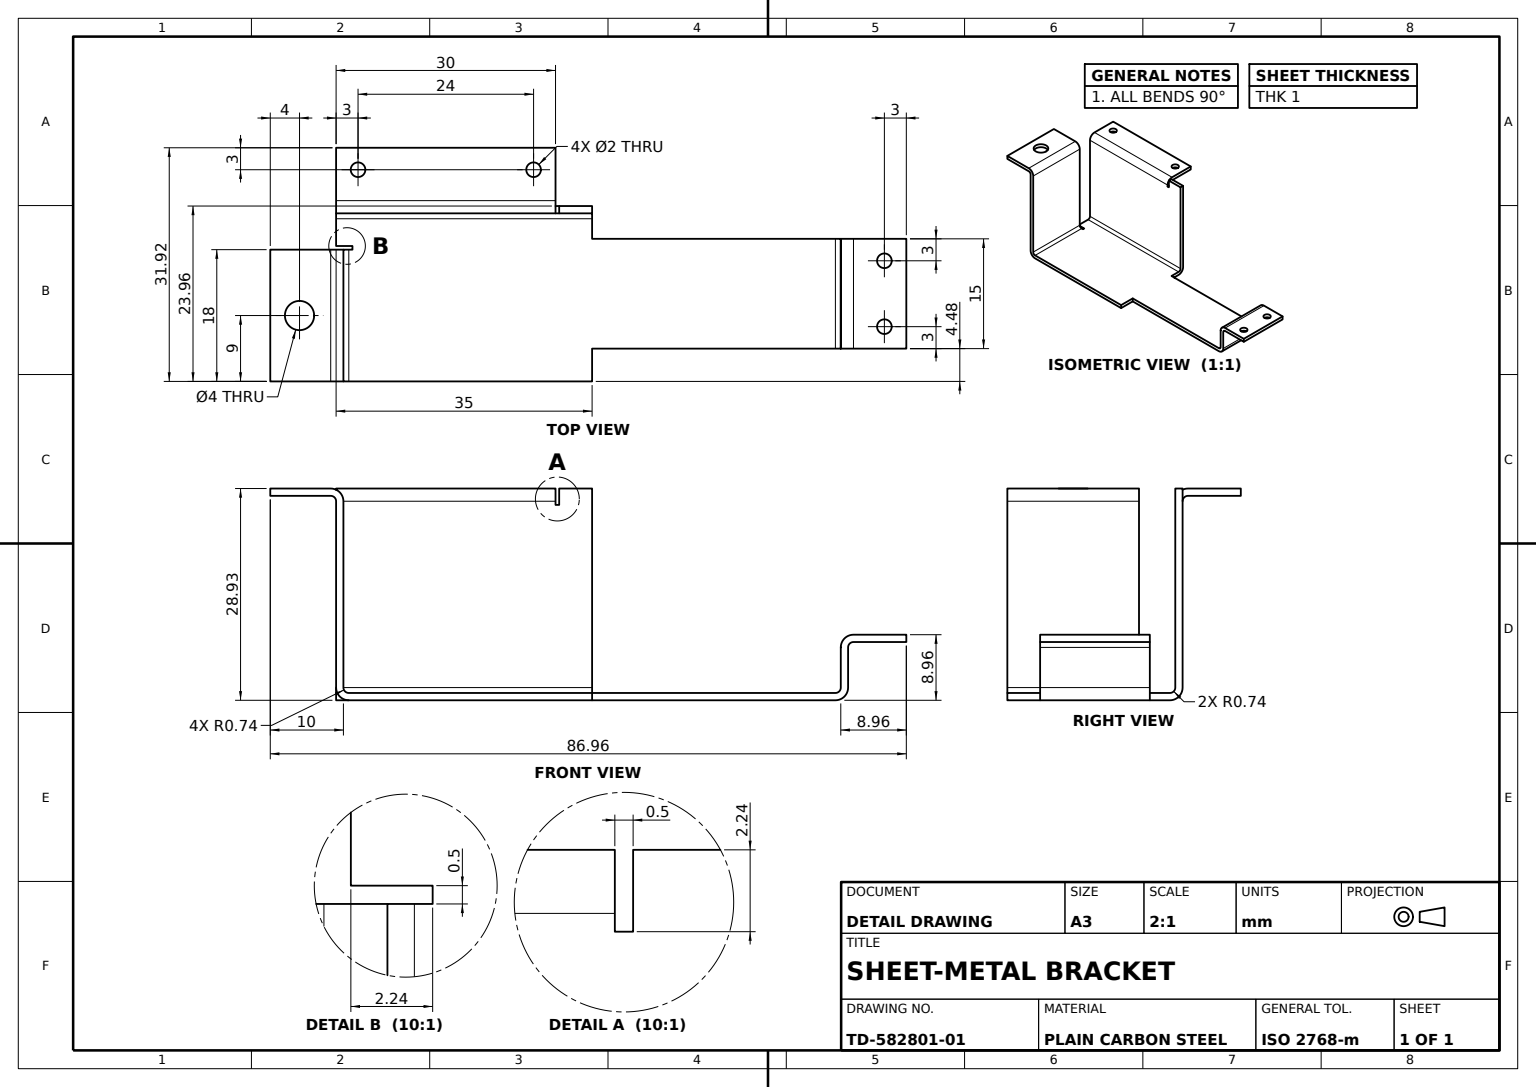
solid
v1 (-4.5,6.96,-58.46)
v2 (-4.5,7.96,-58.46)
e1 v1 v2 LINE
v3 (-4.5,6.96,-56.46)
e2 v1 v3 CIRCLE(AX(P(-4.5,6.96,-57.46),D(0,-1,0),D(0,0,-1)),1)
v4 (-4.5,7.96,-56.46)
e3 v3 v4 LINE
e4 v4 v2 CIRCLE(AX(P(-4.5,7.96,-57.46),D(0,1,0),D(0,0,1)),1)
face CYL(AX(P(-4.5,-2.04,-57.46),D(0,1,0),D(0,0,1)),1) rev [-e1 e2 e3 e4]
v5 (-6.02,27.93,18.2366)
v6 (-6.02,26.1934,16.5)
e5 v5 v6 CIRCLE(AX(P(-6.02,26.1934,18.2366),D(-1,0,0),D(0,0,1)),1.7366)
v7 (11.98,27.93,18.2366)
e6 v7 v5 LINE
v8 (11.98,26.1934,16.5)
e7 v8 v7 CIRCLE(AX(P(11.98,26.1934,18.2366),D(1,0,0),D(0,0,1)),1.7366)
e8 v6 v8 LINE
face CYL(AX(P(-6.02,26.1934,18.2366),D(-1,0,0),D(0,1,0)),1.7366) [-e5 -e6 -e7 -e8]
v9 (-6.02,26.1934,17.5)
v10 (-6.02,0.7366,17.5)
e9 v9 v10 LINE
v11 (11.98,0.7366,17.5)
e10 v11 v10 LINE
v12 (11.98,26.1934,17.5)
e11 v11 v12 LINE
e12 v9 v12 LINE
face PLANE(AX(P(0,0,17.5),D(0,0,-1),D(-1,0,0))) rev [e9 -e10 e11 -e12]
v13 (-10.98,0.7366,-17.5)
v14 (-10.98,0.7366,17.5)
e13 v13 v14 LINE
v15 (-10.98,27.93,-17.5)
e14 v15 v13 LINE
v16 (-10.98,27.93,-13)
e15 v16 v15 LINE
v17 (-10.98,25.6934,-13)
e16 v16 v17 LINE
v18 (-10.98,25.6934,-12.5)
e17 v17 v18 LINE
v19 (-10.98,26.1934,-12.5)
e18 v18 v19 LINE
v20 (-10.98,26.1934,17.5)
e19 v19 v20 LINE
e20 v14 v20 LINE
face PLANE(AX(P(-10.98,0,0),D(1,0,0),D(0,1,0))) [-e13 -e14 -e15 e16 e17 e18 e19 -e20]
v21 (-7.5,7.96,-60.46)
v22 (-7.5,6.96,-60.46)
e21 v21 v22 LINE
v23 (7.5,7.96,-60.46)
e22 v23 v21 LINE
v24 (7.5,6.96,-60.46)
e23 v23 v24 LINE
e24 v24 v22 LINE
face PLANE(AX(P(-7.5,7.96,-60.46),D(0,0,1),D(0,-1,0))) rev [-e21 -e22 e23 e24]
v25 (-7.5,0.7366,-51.5)
v26 (-7.5,0.7366,-52.5)
e25 v25 v26 LINE
v27 (-7.5,6.2234,-51.5)
e26 v25 v27 LINE
v28 (-7.5,6.2234,-52.5)
e27 v28 v27 LINE
e28 v26 v28 LINE
face PLANE(AX(P(-7.5,7.96,-52.5),D(1,0,0),D(0,0,-1))) rev [-e25 e26 -e27 -e28]
e29 v3 v1 CIRCLE(AX(P(-4.5,6.96,-57.46),D(0,-1,0),D(0,0,-1)),1)
e30 v2 v4 CIRCLE(AX(P(-4.5,7.96,-57.46),D(0,1,0),D(0,0,1)),1)
face CYL(AX(P(-4.5,-2.04,-57.46),D(0,1,0),D(0,0,1)),1) rev [e29 e1 e30 -e3]
v29 (11.98,-1,15.7634)
v30 (11.98,-1,-17.5)
e31 v29 v30 LINE
v31 (11.98,0,-17.5)
e32 v30 v31 LINE
v32 (11.98,0,15.7634)
e33 v32 v31 LINE
e34 v32 v29 LINE
face PLANE(AX(P(11.98,-1,17.5),D(1,0,0),D(0,0,-1))) [e31 e32 -e33 e34]
v33 (-6.02,26.93,18.2366)
e35 v33 v5 LINE
v34 (-6.02,26.93,26.5)
e36 v34 v33 LINE
v35 (-6.02,27.93,26.5)
e37 v35 v34 LINE
e38 v35 v5 LINE
face PLANE(AX(P(-6.02,27.93,17.5),D(-1,0,0),D(0,0,1))) [-e35 -e36 -e37 e38]
v36 (-12.7166,26.93,17.5)
v37 (-12.7166,26.93,-12.5)
e39 v36 v37 LINE
v38 (-11.98,26.1934,-12.5)
e40 v37 v38 CIRCLE(AX(P(-12.7166,26.1934,-12.5),D(0,0,-1),D(-1,0,0)),0.7366)
v39 (-11.98,26.1934,17.5)
e41 v38 v39 LINE
e42 v39 v36 CIRCLE(AX(P(-12.7166,26.1934,17.5),D(0,0,1),D(-1,0,0)),0.7366)
face CYL(AX(P(-12.7166,26.1934,-12.5),D(0,0,-1),D(0,1,0)),0.7366) rev [e39 e40 e41 e42]
v40 (11.98,0.7366,16.5)
e43 v40 v8 LINE
e44 v12 v8 LINE
e45 v40 v11 LINE
face PLANE(AX(P(11.98,27.93,17.5),D(-1,0,0),D(0,0,1))) rev [e43 -e44 -e11 -e45]
v41 (-19.94,27.93,-12.5)
v42 (-19.94,27.93,17.5)
e46 v41 v42 LINE
v43 (-19.94,26.93,-12.5)
e47 v41 v43 LINE
v44 (-19.94,26.93,17.5)
e48 v43 v44 LINE
e49 v42 v44 LINE
face PLANE(AX(P(-19.94,27.93,17.5),D(1,0,0),D(0,1,0))) rev [-e46 e47 e48 -e49]
v45 (-7.5,7.96,-53.2366)
e50 v27 v45 CIRCLE(AX(P(-7.5,6.2234,-53.2366),D(-1,0,0),D(0,0,-1)),1.7366)
v46 (7.5,6.2234,-51.5)
e51 v46 v27 LINE
v47 (7.5,7.96,-53.2366)
e52 v47 v46 CIRCLE(AX(P(7.5,6.2234,-53.2366),D(1,0,0),D(0,0,-1)),1.7366)
e53 v47 v45 LINE
face CYL(AX(P(7.5,6.2234,-53.2366),D(1,0,0),D(0,1,0)),1.7366) [-e50 -e51 -e52 e53]
v48 (-7.5,0,-50.7634)
v49 (7.5,0,-50.7634)
e54 v48 v49 LINE
v50 (-7.5,0,-17.5)
e55 v48 v50 LINE
v51 (-10.2434,0,-17.5)
e56 v50 v51 LINE
v52 (-10.2434,0,17.5)
e57 v52 v51 LINE
v53 (-6.52,0,17.5)
e58 v52 v53 LINE
v54 (-6.52,0,15.2634)
e59 v54 v53 LINE
v55 (-6.02,0,15.2634)
e60 v55 v54 LINE
v56 (-6.02,0,15.7634)
e61 v56 v55 LINE
e62 v32 v56 LINE
v57 (7.5,0,-17.5)
e63 v31 v57 LINE
e64 v57 v49 LINE
face PLANE(AX(P(0,0,0),D(0,-1,0),D(0,0,-1))) rev [-e54 e55 e56 -e57 e58 -e59 -e60 -e61 -e62 e33 e63 e64]
v58 (-6.02,0.7366,16.5)
e65 v58 v40 LINE
e66 v6 v58 LINE
face PLANE(AX(P(0,0,16.5),D(0,0,-1),D(-1,0,0))) [-e65 -e66 e8 -e43]
v59 (11.98,26.93,26.5)
e67 v59 v34 LINE
v60 (11.98,27.93,26.5)
e68 v60 v59 LINE
e69 v60 v35 LINE
face PLANE(AX(P(-6.02,27.93,26.5),D(0,0,1),D(0,-1,0))) [-e67 -e68 e69 e37]
v61 (-12.7166,27.93,17.5)
e70 v20 v61 CIRCLE(AX(P(-12.7166,26.1934,17.5),D(0,0,1),D(-1,0,0)),1.7366)
v62 (-12.7166,27.93,-12.5)
e71 v62 v19 CIRCLE(AX(P(-12.7166,26.1934,-12.5),D(0,0,-1),D(-1,0,0)),1.7366)
e72 v62 v61 LINE
face CYL(AX(P(-12.7166,26.1934,-12.5),D(0,0,-1),D(0,1,0)),1.7366) [-e70 -e19 -e71 e72]
v63 (7.5,6.96,-53.2366)
v64 (7.5,6.2234,-52.5)
e73 v63 v64 CIRCLE(AX(P(7.5,6.2234,-53.2366),D(1,0,0),D(0,0,-1)),0.7366)
e74 v63 v47 LINE
e75 v64 v46 LINE
face PLANE(AX(P(7.5,6.2234,-53.2366),D(-1,0,0),D(0,0,1))) rev [-e73 e74 e52 -e75]
v65 (2.98,26.93,20.5)
v66 (2.98,27.93,20.5)
e76 v65 v66 LINE
v67 (2.98,27.93,24.5)
e77 v66 v67 CIRCLE(AX(P(2.98,27.93,22.5),D(0,1,0),D(0,0,1)),2)
v68 (2.98,26.93,24.5)
e78 v68 v67 LINE
e79 v65 v68 CIRCLE(AX(P(2.98,26.93,22.5),D(0,1,0),D(0,0,1)),2)
face CYL(AX(P(2.98,17.93,22.5),D(0,1,0),D(0,0,1)),2) rev [e76 e77 -e78 -e79]
v69 (7.5,0.7366,-51.5)
e80 v69 v25 LINE
e81 v46 v69 LINE
face PLANE(AX(P(0,0,-51.5),D(0,0,1),D(0,-1,0))) [-e26 -e80 -e81 e51]
e82 v14 v52 CIRCLE(AX(P(-10.2434,0.7366,17.5),D(0,0,1),D(1,0,0)),0.7366)
e83 v51 v13 CIRCLE(AX(P(-10.2434,0.7366,-17.5),D(0,0,-1),D(1,0,0)),0.7366)
face CYL(AX(P(-10.2434,0.7366,17.5),D(0,0,1),D(-1,0,0)),0.7366) rev [e13 e82 e57 e83]
e84 v44 v36 LINE
e85 v36 v61 LINE
e86 v42 v61 LINE
face PLANE(AX(P(-11.98,27.93,17.5),D(0,0,-1),D(-1,0,0))) rev [e84 e85 -e86 e49]
v70 (4.5,6.96,-56.46)
v71 (4.5,6.96,-58.46)
e87 v70 v71 CIRCLE(AX(P(4.5,6.96,-57.46),D(0,-1,0),D(0,0,-1)),1)
e88 v71 v70 CIRCLE(AX(P(4.5,6.96,-57.46),D(0,-1,0),D(0,0,-1)),1)
e89 v63 v24 LINE
v72 (-7.5,6.96,-53.2366)
e90 v72 v63 LINE
e91 v22 v72 LINE
face PLANE(AX(P(0,6.96,0),D(0,-1,0),D(0,0,-1))) [-e29 -e2] [-e87 -e88] [-e24 -e89 -e90 -e91]
v73 (-11.98,0.7366,-17.5)
e92 v13 v73 LINE
v74 (-11.98,27.93,-17.5)
e93 v74 v73 LINE
e94 v74 v15 LINE
face PLANE(AX(P(-11.98,0,-17.5),D(0,0,1),D(1,0,0))) rev [e92 -e93 e94 e14]
e95 v62 v41 LINE
e96 v37 v62 LINE
e97 v37 v43 LINE
face PLANE(AX(P(-19.94,27.93,-12.5),D(0,0,1),D(1,0,0))) rev [-e95 -e96 e97 -e47]
e98 v9 v6 LINE
e99 v33 v9 CIRCLE(AX(P(-6.02,26.1934,18.2366),D(-1,0,0),D(0,0,1)),0.7366)
face PLANE(AX(P(-6.02,26.1934,18.2366),D(1,0,0),D(0,0,-1))) rev [-e98 -e99 e35 e5]
e100 v39 v20 LINE
face PLANE(AX(P(-12.7166,26.1934,17.5),D(0,0,1),D(1,0,0))) [-e42 e100 e70 -e85]
e101 v21 v45 LINE
e102 v72 v45 LINE
face PLANE(AX(P(-7.5,7.96,-52.5),D(1,0,0),D(0,0,-1))) rev [-e101 e21 e91 e102]
v75 (4.5,7.96,-58.46)
e103 v71 v75 LINE
v76 (4.5,7.96,-56.46)
e104 v75 v76 CIRCLE(AX(P(4.5,7.96,-57.46),D(0,1,0),D(0,0,1)),1)
e105 v70 v76 LINE
face CYL(AX(P(4.5,-2.04,-57.46),D(0,1,0),D(0,0,1)),1) rev [e103 e104 -e105 e87]
v77 (-11.98,27.93,-13)
v78 (-11.98,25.6934,-13)
e106 v77 v78 LINE
e107 v78 v17 LINE
e108 v77 v16 LINE
face PLANE(AX(P(-11.98,27.93,-13),D(0,0,1),D(1,0,0))) [e106 e107 -e16 -e108]
e109 v11 v29 CIRCLE(AX(P(11.98,0.7366,15.7634),D(1,0,0),D(0,0,-1)),1.7366)
v79 (-6.02,-1,15.7634)
e110 v79 v10 CIRCLE(AX(P(-6.02,0.7366,15.7634),D(-1,0,0),D(0,0,-1)),1.7366)
e111 v29 v79 LINE
face CYL(AX(P(11.98,0.7366,15.7634),D(1,0,0),D(0,0,1)),1.7366) [-e109 e10 -e110 -e111]
v80 (-11.98,0.7366,17.5)
e112 v14 v80 LINE
e113 v80 v39 LINE
face PLANE(AX(P(-11.98,27.93,17.5),D(0,0,-1),D(-1,0,0))) rev [-e112 e20 -e100 -e113]
v81 (-16.94,27.93,-8.5)
v82 (-16.94,27.93,-10.5)
e114 v81 v82 CIRCLE(AX(P(-16.94,27.93,-9.5),D(0,1,0),D(0,0,1)),1)
v83 (-16.94,26.93,-10.5)
e115 v83 v82 LINE
v84 (-16.94,26.93,-8.5)
e116 v83 v84 CIRCLE(AX(P(-16.94,26.93,-9.5),D(0,-1,0),D(0,0,-1)),1)
e117 v84 v81 LINE
face CYL(AX(P(-16.94,17.93,-9.5),D(0,1,0),D(0,0,1)),1) rev [e114 -e115 e116 e117]
e118 v25 v48 CIRCLE(AX(P(-7.5,0.7366,-50.7634),D(-1,0,0),D(0,0,1)),0.7366)
v85 (-7.5,-1,-50.7634)
e119 v26 v85 CIRCLE(AX(P(-7.5,0.7366,-50.7634),D(-1,0,0),D(0,0,1)),1.7366)
e120 v48 v85 LINE
face PLANE(AX(P(-7.5,0.7366,-50.7634),D(1,0,0),D(0,0,-1))) rev [-e118 e25 e119 -e120]
e121 v77 v74 LINE
face PLANE(AX(P(-11.98,27.93,-17.5),D(0,-1,0),D(1,0,0))) rev [-e94 -e121 e108 e15]
v86 (7.5,-1,-17.5)
e122 v86 v57 LINE
e123 v30 v86 LINE
face PLANE(AX(P(-11.98,-1,-17.5),D(0,0,-1),D(-1,0,0))) [e122 -e63 -e32 e123]
e124 v47 v23 LINE
e125 v76 v75 CIRCLE(AX(P(4.5,7.96,-57.46),D(0,1,0),D(0,0,1)),1)
face PLANE(AX(P(0,7.96,0),D(0,-1,0),D(0,0,-1))) rev [e124 e22 e101 -e53] [-e125 -e104] [-e30 -e4]
v87 (-6.02,-1,15.2634)
e126 v79 v87 LINE
v88 (-6.52,-1,15.2634)
e127 v87 v88 LINE
v89 (-6.52,-1,17.5)
e128 v88 v89 LINE
v90 (-10.2434,-1,17.5)
e129 v90 v89 LINE
v91 (-10.2434,-1,-17.5)
e130 v90 v91 LINE
v92 (-7.5,-1,-17.5)
e131 v92 v91 LINE
e132 v85 v92 LINE
v93 (7.5,-1,-50.7634)
e133 v85 v93 LINE
e134 v86 v93 LINE
face PLANE(AX(P(0,-1,0),D(0,-1,0),D(0,0,-1))) [e111 e126 e127 e128 -e129 e130 -e131 -e132 e133 -e134 -e123 -e31]
v94 (11.98,26.93,18.2366)
e135 v94 v7 LINE
e136 v12 v94 CIRCLE(AX(P(11.98,26.1934,18.2366),D(1,0,0),D(0,0,1)),0.7366)
face PLANE(AX(P(11.98,26.1934,18.2366),D(1,0,0),D(0,0,-1))) [e7 -e135 -e136 e44]
e137 v7 v60 LINE
e138 v94 v59 LINE
face PLANE(AX(P(11.98,27.93,26.5),D(1,0,0),D(0,0,-1))) [e135 e137 e68 -e138]
e139 v38 v19 LINE
face PLANE(AX(P(-12.7166,26.1934,-12.5),D(0,0,1),D(1,0,0))) rev [-e139 -e40 e96 e71]
v95 (-16.94,26.93,15.5)
v96 (-16.94,27.93,15.5)
e140 v95 v96 LINE
v97 (-16.94,27.93,13.5)
e141 v96 v97 CIRCLE(AX(P(-16.94,27.93,14.5),D(0,1,0),D(0,0,1)),1)
v98 (-16.94,26.93,13.5)
e142 v98 v97 LINE
e143 v98 v95 CIRCLE(AX(P(-16.94,26.93,14.5),D(0,-1,0),D(0,0,-1)),1)
face CYL(AX(P(-16.94,17.93,14.5),D(0,1,0),D(0,0,1)),1) rev [e140 e141 -e142 e143]
v99 (7.5,0.7366,-52.5)
e144 v26 v99 LINE
e145 v93 v99 CIRCLE(AX(P(7.5,0.7366,-50.7634),D(1,0,0),D(0,0,1)),1.7366)
face CYL(AX(P(-7.5,0.7366,-50.7634),D(-1,0,0),D(0,0,-1)),1.7366) [-e119 e144 -e145 -e133]
e146 v67 v66 CIRCLE(AX(P(2.98,27.93,22.5),D(0,1,0),D(0,0,1)),2)
face PLANE(AX(P(0,27.93,0),D(0,1,0),D(0,0,1))) [-e38 -e69 -e137 e6] [-e77 -e146]
e147 v58 v10 LINE
face PLANE(AX(P(-6.02,0,17.5),D(1,0,0),D(0,0,-1))) rev [e147 -e9 e98 e66]
e148 v68 v65 CIRCLE(AX(P(2.98,26.93,22.5),D(0,1,0),D(0,0,1)),2)
face CYL(AX(P(2.98,17.93,22.5),D(0,1,0),D(0,0,1)),2) rev [-e148 e78 e146 -e76]
e149 v52 v90 LINE
e150 v80 v90 CIRCLE(AX(P(-10.2434,0.7366,17.5),D(0,0,1),D(1,0,0)),1.7366)
face PLANE(AX(P(-10.2434,0.7366,17.5),D(0,0,-1),D(-1,0,0))) rev [-e149 -e82 e112 e150]
e151 v92 v50 LINE
face PLANE(AX(P(-7.5,-1,-17.5),D(-1,0,0),D(0,0,1))) [e120 e132 e151 -e55]
e152 v84 v83 CIRCLE(AX(P(-16.94,26.93,-9.5),D(0,-1,0),D(0,0,-1)),1)
e153 v95 v98 CIRCLE(AX(P(-16.94,26.93,14.5),D(0,-1,0),D(0,0,-1)),1)
face PLANE(AX(P(0,26.93,0),D(0,-1,0),D(0,0,-1))) [-e152 -e116] [-e153 -e143] [-e97 -e39 -e84 -e48]
e154 v53 v89 LINE
face PLANE(AX(P(-11.98,-1,17.5),D(0,0,1),D(1,0,0))) [e129 -e154 -e58 e149]
e155 v91 v73 CIRCLE(AX(P(-10.2434,0.7366,-17.5),D(0,0,-1),D(1,0,0)),1.7366)
e156 v80 v73 LINE
face CYL(AX(P(-10.2434,0.7366,17.5),D(0,0,1),D(-1,0,0)),1.7366) [-e155 -e130 -e150 e156]
e157 v56 v79 LINE
e158 v56 v58 CIRCLE(AX(P(-6.02,0.7366,15.7634),D(-1,0,0),D(0,0,-1)),0.7366)
face PLANE(AX(P(-6.02,0.7366,15.7634),D(-1,0,0),D(0,0,1))) [e157 e110 -e147 -e158]
e159 v94 v33 LINE
face PLANE(AX(P(0,26.93,0),D(0,1,0),D(0,0,1))) rev [e79 e148] [-e159 e138 e67 e36]
e160 v49 v93 LINE
face PLANE(AX(P(7.5,-1,-17.5),D(1,0,0),D(0,0,-1))) [-e122 e134 -e160 -e64]
v100 (-11.98,25.6934,-12.5)
e161 v100 v18 LINE
e162 v100 v38 LINE
face PLANE(AX(P(-11.98,25.6934,-12.5),D(0,0,-1),D(-1,0,0))) [-e18 -e161 e162 e139]
e163 v78 v100 LINE
face PLANE(AX(P(-11.98,0,0),D(1,0,0),D(0,1,0))) rev [e113 -e41 -e162 -e163 -e106 e121 e93 -e156]
e164 v40 v32 CIRCLE(AX(P(11.98,0.7366,15.7634),D(1,0,0),D(0,0,-1)),0.7366)
face CYL(AX(P(11.98,0.7366,15.7634),D(1,0,0),D(0,0,1)),0.7366) rev [e62 e158 e65 e164]
face PLANE(AX(P(11.98,0.7366,15.7634),D(-1,0,0),D(0,0,1))) rev [-e34 -e164 e45 e109]
e165 v69 v99 LINE
e166 v64 v99 LINE
face PLANE(AX(P(7.5,0,-52.5),D(-1,0,0),D(0,0,1))) rev [e165 -e166 e75 e81]
face CYL(AX(P(4.5,-2.04,-57.46),D(0,1,0),D(0,0,1)),1) rev [e88 e105 e125 -e103]
e167 v28 v72 CIRCLE(AX(P(-7.5,6.2234,-53.2366),D(-1,0,0),D(0,0,-1)),0.7366)
face PLANE(AX(P(-7.5,6.2234,-53.2366),D(-1,0,0),D(0,0,1))) [-e167 e27 e50 -e102]
e168 v82 v81 CIRCLE(AX(P(-16.94,27.93,-9.5),D(0,1,0),D(0,0,1)),1)
face CYL(AX(P(-16.94,17.93,-9.5),D(0,1,0),D(0,0,1)),1) rev [-e117 e152 e115 e168]
e169 v51 v91 LINE
face PLANE(AX(P(-10.2434,0.7366,-17.5),D(0,0,-1),D(-1,0,0))) [-e92 -e83 e169 e155]
e170 v55 v87 LINE
e171 v54 v88 LINE
face PLANE(AX(P(-6.02,0,15.2634),D(0,0,1),D(0,-1,0))) [-e170 e60 e171 -e127]
e172 v64 v28 LINE
face PLANE(AX(P(0,0,-52.5),D(0,0,1),D(0,-1,0))) rev [-e172 e166 -e144 e28]
face PLANE(AX(P(-11.98,25.6934,-13),D(0,1,0),D(-1,0,0))) [-e107 e163 e161 -e17]
face PLANE(AX(P(7.5,7.96,-60.46),D(-1,0,0),D(0,0,1))) rev [e89 -e23 -e124 -e74]
e173 v49 v69 CIRCLE(AX(P(7.5,0.7366,-50.7634),D(1,0,0),D(0,0,1)),0.7366)
face PLANE(AX(P(7.5,0.7366,-50.7634),D(1,0,0),D(0,0,-1))) [e160 e145 -e165 -e173]
e174 v97 v96 CIRCLE(AX(P(-16.94,27.93,14.5),D(0,1,0),D(0,0,1)),1)
face PLANE(AX(P(0,27.93,0),D(0,-1,0),D(0,0,-1))) rev [-e114 -e168] [-e141 -e174] [e95 e46 e86 -e72]
face PLANE(AX(P(-6.02,0,15.7634),D(-1,0,0),D(0,0,1))) [-e157 e61 e170 -e126]
face CYL(AX(P(-7.5,0.7366,-50.7634),D(-1,0,0),D(0,0,-1)),0.7366) rev [e80 e118 e54 e173]
face CYL(AX(P(-16.94,17.93,14.5),D(0,1,0),D(0,0,1)),1) rev [-e140 e153 e142 e174]
face CYL(AX(P(7.5,6.2234,-53.2366),D(1,0,0),D(0,1,0)),0.7366) rev [e90 e73 e172 e167]
face PLANE(AX(P(-6.52,0,15.2634),D(1,0,0),D(0,0,-1))) [-e171 e59 e154 -e128]
face PLANE(AX(P(-11.98,-1,-17.5),D(0,0,-1),D(-1,0,0))) [-e169 -e56 -e151 e131]
face CYL(AX(P(-6.02,26.1934,18.2366),D(-1,0,0),D(0,1,0)),0.7366) rev [e136 e159 e99 e12]
